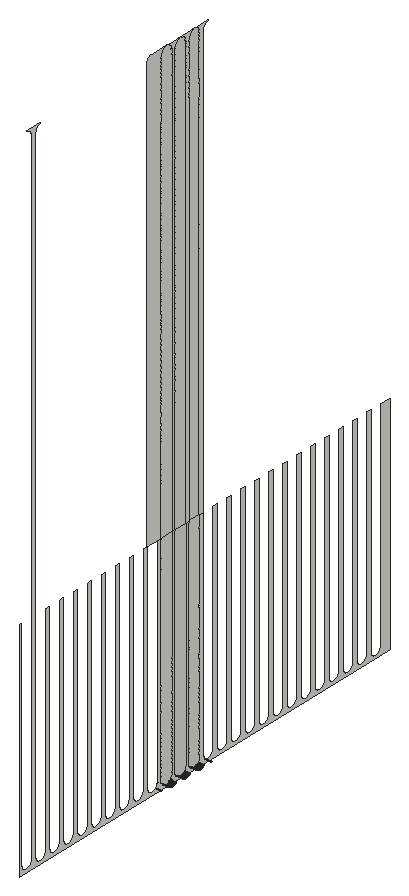
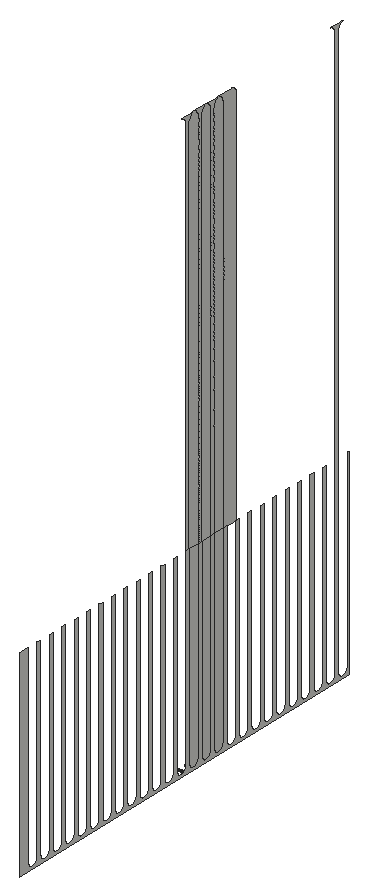
# SketchUp Ruby script. Lengths in inches.
U = 1.inch
M = Sketchup.active_model
def pt(a) = Geom::Point3d.new(a.map { |v| v * U })
def face(e, loops, mat)
  f = e.add_face(loops[0].map { |a| pt(a) })
  loops[1..].each { |l| e.add_face(l.map { |a| pt(a) }).erase! }
  f.material = f.back_material = mat if mat
  f
end
# faces: each face lists its corners as indices into pts; further lists are holes
def faces(e, pts, list, mat = nil) = list.each { |f| face(e, (f[0].is_a?(Array) ? f : [f]).map { |l| l.map { |i| pts[i] } }, mat) }
# xy, xz, yz: faces in a plane at the given z, y or x. An outline is a flat list of corners, or four numbers for a rectangle; further outlines are holes
def ring(l) = l.size == 4 ? [[l[0], l[1]], [l[2], l[1]], [l[2], l[3]], [l[0], l[3]]] : l.each_slice(2).to_a
def flat(e, list, mat, &to3) = list.each { |f| face(e, (f[0].is_a?(Array) ? f : [f]).map { |l| ring(l).map { |u, v| to3.(u, v) } }, mat) }
def xy(e, z, list, mat = nil) = flat(e, list, mat) { |x, y| [x, y, z] }
def xz(e, y, list, mat = nil) = flat(e, list, mat) { |x, z| [x, y, z] }
def yz(e, x, list, mat = nil) = flat(e, list, mat) { |y, z| [x, y, z] }
def lines(e, pts, list) = list.each { |a, b| e.add_line(pt(pts[a]), pt(pts[b])) }
# prism: a flat outline (further loops are holes) pulled along v
def prism(e, loops, v, mat = nil)
  f = face(e, loops, mat); d = Geom::Vector3d.new(v.map { |x| x * U })
  f.pushpull(f.normal.samedirection?(d) ? d.length : -d.length)
end
def box(e, o, s, mat = nil) = prism(e, [[o, [o[0] + s[0], o[1], o[2]], [o[0] + s[0], o[1] + s[1], o[2]], [o[0], o[1] + s[1], o[2]]]], [0, 0, s[2]], mat)
def at(x, y, z, deg = 0) = Geom::Transformation.translation(pt([x, y, z])) * Geom::Transformation.rotation(ORIGIN, Z_AXIS, deg.degrees)
def axes(o, x, y, z) = Geom::Transformation.new([*x, 0, *y, 0, *z, 0, *pt(o).to_a, 1])
def part(name) = M.definitions.add(name)
# library, detail: a bought-in or finely detailed component or shape, given as its bounding box
def library(name, o, s) = part(name).tap { |d| box(d.entities, o, s) }
def detail(e, o, s) = box(e.add_group.entities, o, s)
def put(e, d, t, mat = nil) = e.add_instance(d, t).tap { |i| i.material = mat if mat }
def group(e, t, mat = nil) = e.add_group.tap { |g| g.transformation = t; g.material = mat if mat }.entities
root = M.entities
yz(root,9,[[15,2,88.732,2,88.732,38,87,38,87,3.521,87.003,3.464,87.003,3.407,87,3.363,86.993,3.292,86.983,3.236,86.97,3.18,86.954,3.125,86.936,3.071,86.914,3.018,86.889,2.966,86.862,2.915,86.831,2.867,86.799,2.82,86.763,2.774,86.726,2.731,86.685,2.69,86.643,2.651,86.599,2.615,86.553,2.581,86.504,2.55,86.455,2.521,86.404,2.495,86.351,2.473,86.297,2.452,86.242,2.435,86.187,2.421,86.131,2.41,86.074,2.403,86.017,2.398,85.959,2.396,85.902,2.398,85.845,2.403,85.788,2.41,85.732,2.421,85.676,2.435,85.621,2.452,85.568,2.473,85.515,2.495,85.464,2.521,85.414,2.55,85.366,2.581,85.32,2.615,85.275,2.651,85.233,2.69,85.193,2.731,85.155,2.774,85.12,2.82,85.087,2.867,85.057,2.915,85.029,2.966,85.005,3.018,84.983,3.071,84.964,3.125,84.948,3.18,84.936,3.236,84.926,3.292,84.918,3.363,84.916,3.407,84.916,3.464,84.918,3.521,84.918,38,84.212,38,84.212,3.521,84.215,3.464,84.215,3.407,84.212,3.363,84.205,3.292,84.195,3.236,84.183,3.18,84.167,3.125,84.148,3.071,84.126,3.018,84.102,2.966,84.074,2.915,84.044,2.867,84.011,2.82,83.976,2.774,83.938,2.731,83.898,2.69,83.856,2.651,83.811,2.615,83.765,2.581,83.717,2.55,83.667,2.521,83.616,2.495,83.563,2.473,83.51,2.452,83.455,2.435,83.399,2.421,83.343,2.41,83.286,2.403,83.229,2.398,83.172,2.396,83.114,2.398,83.057,2.403,83,2.41,82.944,2.421,82.889,2.435,82.834,2.452,82.78,2.473,82.727,2.495,82.676,2.521,82.627,2.55,82.578,2.581,82.532,2.615,82.488,2.651,82.446,2.69,82.405,2.731,82.368,2.774,82.332,2.82,82.3,2.867,82.269,2.915,82.242,2.966,82.217,3.018,82.195,3.071,82.177,3.125,82.161,3.18,82.148,3.236,82.138,3.292,82.131,3.363,82.128,3.407,82.128,3.464,82.131,3.521,82.131,38,81.425,38,81.425,3.521,81.428,3.464,81.428,3.407,81.425,3.363,81.418,3.292,81.408,3.236,81.395,3.18,81.379,3.125,81.361,3.071,81.339,3.018,81.314,2.966,81.287,2.915,81.256,2.867,81.224,2.82,81.188,2.774,81.151,2.731,81.11,2.69,81.068,2.651,81.024,2.615,80.978,2.581,80.929,2.55,80.88,2.521,80.829,2.495,80.776,2.473,80.722,2.452,80.667,2.435,80.612,2.421,80.556,2.41,80.499,2.403,80.442,2.398,80.384,2.396,80.327,2.398,80.27,2.403,80.213,2.41,80.157,2.421,80.101,2.435,80.046,2.452,79.993,2.473,79.94,2.495,79.889,2.521,79.839,2.55,79.791,2.581,79.745,2.615,79.7,2.651,79.658,2.69,79.618,2.731,79.58,2.774,79.545,2.82,79.512,2.867,79.482,2.915,79.454,2.966,79.43,3.018,79.408,3.071,79.389,3.125,79.373,3.18,79.361,3.236,79.351,3.292,79.343,3.363,79.341,3.407,79.341,3.464,79.343,3.521,79.343,38,78.637,38,78.637,3.521,78.64,3.464,78.64,3.407,78.637,3.363,78.63,3.292,78.62,3.236,78.608,3.18,78.592,3.125,78.573,3.071,78.551,3.018,78.527,2.966,78.499,2.915,78.469,2.867,78.436,2.82,78.401,2.774,78.363,2.731,78.323,2.69,78.281,2.651,78.236,2.615,78.19,2.581,78.142,2.55,78.092,2.521,78.041,2.495,77.988,2.473,77.935,2.452,77.88,2.435,77.824,2.421,77.768,2.41,77.711,2.403,77.654,2.398,77.597,2.396,77.539,2.398,77.482,2.403,77.425,2.41,77.369,2.421,77.314,2.435,77.259,2.452,77.205,2.473,77.152,2.495,77.101,2.521,77.052,2.55,77.003,2.581,76.957,2.615,76.913,2.651,76.871,2.69,76.83,2.731,76.793,2.774,76.757,2.82,76.725,2.867,76.694,2.915,76.667,2.966,76.642,3.018,76.62,3.071,76.602,3.125,76.586,3.18,76.573,3.236,76.563,3.292,76.556,3.363,76.553,3.407,76.553,3.464,76.556,3.521,76.556,38,75.85,38,75.85,3.521,75.853,3.464,75.853,3.407,75.85,3.363,75.843,3.292,75.833,3.236,75.82,3.18,75.804,3.125,75.786,3.071,75.764,3.018,75.739,2.966,75.712,2.915,75.681,2.867,75.649,2.82,75.613,2.774,75.576,2.731,75.535,2.69,75.493,2.651,75.449,2.615,75.403,2.581,75.354,2.55,75.305,2.521,75.254,2.495,75.201,2.473,75.147,2.452,75.092,2.435,75.037,2.421,74.981,2.41,74.924,2.403,74.867,2.398,74.809,2.396,74.752,2.398,74.695,2.403,74.638,2.41,74.582,2.421,74.526,2.435,74.471,2.452,74.418,2.473,74.365,2.495,74.314,2.521,74.264,2.55,74.216,2.581,74.17,2.615,74.125,2.651,74.083,2.69,74.043,2.731,74.005,2.774,73.97,2.82,73.937,2.867,73.907,2.915,73.879,2.966,73.855,3.018,73.833,3.071,73.814,3.125,73.798,3.18,73.786,3.236,73.776,3.292,73.768,3.363,73.766,3.407,73.766,3.464,73.768,3.521,73.768,38,73.0625,38,73.0625,3.521,73.065,3.464,73.065,3.407,73.0625,3.363,73.055,3.292,73.045,3.236,73.033,3.18,73.017,3.125,72.998,3.071,72.976,3.018,72.952,2.966,72.924,2.915,72.894,2.867,72.861,2.82,72.826,2.774,72.788,2.731,72.748,2.69,72.706,2.651,72.661,2.615,72.615,2.581,72.567,2.55,72.517,2.521,72.466,2.495,72.413,2.473,72.36,2.452,72.305,2.435,72.249,2.421,72.193,2.41,72.136,2.403,72.079,2.398,72.022,2.396,71.964,2.398,71.907,2.403,71.85,2.41,71.794,2.421,71.739,2.435,71.684,2.452,71.63,2.473,71.577,2.495,71.526,2.521,71.477,2.55,71.428,2.581,71.382,2.615,71.338,2.651,71.296,2.69,71.255,2.731,71.218,2.774,71.182,2.82,71.15,2.867,71.119,2.915,71.092,2.966,71.067,3.018,71.045,3.071,71.027,3.125,71.011,3.18,70.998,3.236,70.988,3.292,70.981,3.363,70.978,3.407,70.978,3.464,70.981,3.521,70.981,38,70.275,38,70.275,3.521,70.278,3.464,70.278,3.407,70.275,3.363,70.268,3.292,70.258,3.236,70.245,3.18,70.229,3.125,70.211,3.071,70.189,3.018,70.164,2.966,70.137,2.915,70.106,2.867,70.074,2.82,70.038,2.774,70.001,2.731,69.96,2.69,69.918,2.651,69.874,2.615,69.828,2.581,69.779,2.55,69.73,2.521,69.679,2.495,69.626,2.473,69.572,2.452,69.517,2.435,69.462,2.421,69.406,2.41,69.349,2.403,69.292,2.398,69.234,2.396,69.177,2.398,69.12,2.403,69.063,2.41,69.007,2.421,68.951,2.435,68.896,2.452,68.843,2.473,68.79,2.495,68.739,2.521,68.689,2.55,68.641,2.581,68.595,2.615,68.55,2.651,68.508,2.69,68.468,2.731,68.43,2.774,68.395,2.82,68.362,2.867,68.332,2.915,68.304,2.966,68.28,3.018,68.258,3.071,68.239,3.125,68.223,3.18,68.211,3.236,68.201,3.292,68.193,3.363,68.191,3.407,68.191,3.464,68.193,3.521,68.193,38,67.487,38,67.487,3.521,67.49,3.464,67.49,3.407,67.487,3.363,67.48,3.292,67.47,3.236,67.458,3.18,67.442,3.125,67.423,3.071,67.401,3.018,67.377,2.966,67.349,2.915,67.319,2.867,67.286,2.82,67.251,2.774,67.213,2.731,67.173,2.69,67.131,2.651,67.086,2.615,67.04,2.581,66.992,2.55,66.942,2.521,66.891,2.495,66.838,2.473,66.785,2.452,66.73,2.435,66.674,2.421,66.618,2.41,66.561,2.403,66.504,2.398,66.447,2.396,66.389,2.398,66.332,2.403,66.275,2.41,66.219,2.421,66.164,2.435,66.109,2.452,66.055,2.473,66.002,2.495,65.951,2.521,65.902,2.55,65.853,2.581,65.807,2.615,65.763,2.651,65.721,2.69,65.68,2.731,65.643,2.774,65.607,2.82,65.575,2.867,65.544,2.915,65.517,2.966,65.492,3.018,65.47,3.071,65.452,3.125,65.436,3.18,65.423,3.236,65.413,3.292,65.406,3.363,65.403,3.407,65.403,3.464,65.406,3.521,65.406,38,64.7,38,64.7,3.521,64.703,3.464,64.703,3.407,64.7,3.363,64.693,3.292,64.683,3.236,64.67,3.18,64.654,3.125,64.636,3.071,64.614,3.018,64.589,2.966,64.562,2.915,64.531,2.867,64.499,2.82,64.463,2.774,64.426,2.731,64.385,2.69,64.343,2.651,64.299,2.615,64.253,2.581,64.204,2.55,64.155,2.521,64.104,2.495,64.051,2.473,63.997,2.452,63.942,2.435,63.887,2.421,63.831,2.41,63.774,2.403,63.717,2.398,63.659,2.396,63.602,2.398,63.545,2.403,63.488,2.41,63.432,2.421,63.376,2.435,63.321,2.452,63.268,2.473,63.215,2.495,63.164,2.521,63.114,2.55,63.066,2.581,63.02,2.615,62.975,2.651,62.933,2.69,62.893,2.731,62.855,2.774,62.82,2.82,62.787,2.867,62.757,2.915,62.729,2.966,62.705,3.018,62.683,3.071,62.664,3.125,62.648,3.18,62.636,3.236,62.626,3.292,62.618,3.363,62.616,3.407,62.616,3.464,62.618,3.521,62.618,38,61.912,38,61.912,3.521,61.915,3.464,61.915,3.407,61.912,3.363,61.905,3.292,61.895,3.236,61.883,3.18,61.867,3.125,61.848,3.071,61.826,3.018,61.802,2.966,61.774,2.915,61.744,2.867,61.711,2.82,61.676,2.774,61.638,2.731,61.598,2.69,61.556,2.651,61.511,2.615,61.465,2.581,61.417,2.55,61.367,2.521,61.316,2.495,61.263,2.473,61.21,2.452,61.155,2.435,61.099,2.421,61.043,2.41,60.986,2.403,60.929,2.398,60.872,2.396,60.814,2.398,60.757,2.403,60.7,2.41,60.644,2.421,60.589,2.435,60.534,2.452,60.48,2.473,60.427,2.495,60.376,2.521,60.327,2.55,60.278,2.581,60.232,2.615,60.188,2.651,60.146,2.69,60.105,2.731,60.068,2.774,60.032,2.82,60,2.867,59.969,2.915,59.942,2.966,59.917,3.018,59.895,3.071,59.877,3.125,59.861,3.18,59.848,3.236,59.838,3.292,59.831,3.363,59.828,3.407,59.828,3.464,59.831,3.521,59.831,38,59.125,38,59.125,3.521,59.128,3.464,59.128,3.407,59.125,3.363,59.118,3.292,59.108,3.236,59.095,3.18,59.079,3.125,59.061,3.071,59.039,3.018,59.014,2.966,58.987,2.915,58.956,2.867,58.924,2.82,58.888,2.774,58.851,2.731,58.81,2.69,58.768,2.651,58.724,2.615,58.678,2.581,58.629,2.55,58.58,2.521,58.529,2.495,58.476,2.473,58.422,2.452,58.367,2.435,58.312,2.421,58.256,2.41,58.199,2.403,58.142,2.398,58.084,2.396,58.027,2.398,57.97,2.403,57.913,2.41,57.857,2.421,57.801,2.435,57.746,2.452,57.693,2.473,57.64,2.495,57.589,2.521,57.539,2.55,57.491,2.581,57.445,2.615,57.4,2.651,57.358,2.69,57.318,2.731,57.28,2.774,57.245,2.82,57.212,2.867,57.182,2.915,57.154,2.966,57.13,3.018,57.108,3.071,57.089,3.125,57.073,3.18,57.061,3.236,57.051,3.292,57.043,3.363,57.041,3.407,57.041,3.464,57.043,3.521,57.043,38,56.338,38,56.338,3.521,56.34,3.464,56.34,3.407,56.338,3.363,56.33,3.292,56.32,3.236,56.308,3.18,56.292,3.125,56.273,3.071,56.251,3.018,56.227,2.966,56.199,2.915,56.169,2.867,56.136,2.82,56.101,2.774,56.063,2.731,56.023,2.69,55.981,2.651,55.936,2.615,55.89,2.581,55.842,2.55,55.792,2.521,55.741,2.495,55.688,2.473,55.635,2.452,55.58,2.435,55.524,2.421,55.468,2.41,55.411,2.403,55.354,2.398,55.297,2.396,55.239,2.398,55.182,2.403,55.125,2.41,55.069,2.421,55.014,2.435,54.959,2.452,54.905,2.473,54.852,2.495,54.801,2.521,54.752,2.55,54.703,2.581,54.657,2.615,54.613,2.651,54.571,2.69,54.53,2.731,54.493,2.774,54.457,2.82,54.425,2.867,54.394,2.915,54.367,2.966,54.342,3.018,54.32,3.071,54.302,3.125,54.286,3.18,54.273,3.236,54.263,3.292,54.256,3.363,54.253,3.407,54.253,3.464,54.256,3.521,54.256,38,53.55,38,53.55,3.521,53.553,3.464,53.553,3.407,53.55,3.363,53.543,3.292,53.533,3.236,53.52,3.18,53.504,3.125,53.486,3.071,53.464,3.018,53.439,2.966,53.412,2.915,53.381,2.867,53.349,2.82,53.313,2.774,53.276,2.731,53.235,2.69,53.193,2.651,53.149,2.615,53.103,2.581,53.054,2.55,53.005,2.521,52.954,2.495,52.901,2.473,52.847,2.452,52.792,2.435,52.737,2.421,52.681,2.41,52.624,2.403,52.567,2.398,52.509,2.396,52.452,2.398,52.395,2.403,52.338,2.41,52.282,2.421,52.226,2.435,52.171,2.452,52.118,2.473,52.065,2.495,52.014,2.521,51.964,2.55,51.916,2.581,51.87,2.615,51.825,2.651,51.783,2.69,51.743,2.731,51.705,2.774,51.67,2.82,51.637,2.867,51.607,2.915,51.579,2.966,51.555,3.018,51.533,3.071,51.514,3.125,51.498,3.18,51.486,3.236,51.476,3.292,51.468,3.363,51.466,3.407,51.466,3.464,51.468,3.521,51.468,38,50.762,38,50.762,3.521,50.765,3.464,50.765,3.407,50.762,3.363,50.755,3.292,50.745,3.236,50.733,3.18,50.717,3.125,50.698,3.071,50.676,3.018,50.652,2.966,50.624,2.915,50.594,2.867,50.561,2.82,50.526,2.774,50.488,2.731,50.448,2.69,50.406,2.651,50.361,2.615,50.315,2.581,50.267,2.55,50.217,2.521,50.166,2.495,50.113,2.473,50.06,2.452,50.005,2.435,49.949,2.421,49.893,2.41,49.836,2.403,49.779,2.398,49.722,2.396,49.664,2.398,49.607,2.403,49.55,2.41,49.494,2.421,49.439,2.435,49.384,2.452,49.33,2.473,49.277,2.495,49.226,2.521,49.177,2.55,49.128,2.581,49.082,2.615,49.038,2.651,48.996,2.69,48.955,2.731,48.918,2.774,48.882,2.82,48.85,2.867,48.819,2.915,48.792,2.966,48.767,3.018,48.745,3.071,48.727,3.125,48.711,3.18,48.698,3.236,48.688,3.292,48.681,3.363,48.678,3.407,48.678,3.464,48.681,3.521,48.681,38,47.975,38,47.975,3.521,47.978,3.464,47.978,3.407,47.975,3.363,47.968,3.292,47.958,3.236,47.945,3.18,47.929,3.125,47.911,3.071,47.889,3.018,47.864,2.966,47.837,2.915,47.806,2.867,47.774,2.82,47.738,2.774,47.701,2.731,47.66,2.69,47.618,2.651,47.574,2.615,47.528,2.581,47.479,2.55,47.43,2.521,47.379,2.495,47.326,2.473,47.272,2.452,47.217,2.435,47.162,2.421,47.106,2.41,47.049,2.403,46.992,2.398,46.934,2.396,46.877,2.398,46.82,2.403,46.763,2.41,46.707,2.421,46.651,2.435,46.596,2.452,46.543,2.473,46.49,2.495,46.439,2.521,46.389,2.55,46.341,2.581,46.295,2.615,46.25,2.651,46.208,2.69,46.168,2.731,46.13,2.774,46.095,2.82,46.062,2.867,46.032,2.915,46.004,2.966,45.98,3.018,45.958,3.071,45.939,3.125,45.923,3.18,45.911,3.236,45.901,3.292,45.893,3.363,45.891,3.407,45.891,3.464,45.893,3.521,45.893,38,45.1875,38,45.1875,3.521,45.19,3.464,45.19,3.407,45.1875,3.363,45.18,3.292,45.17,3.236,45.158,3.18,45.142,3.125,45.123,3.071,45.101,3.018,45.077,2.966,45.049,2.915,45.019,2.867,44.986,2.82,44.951,2.774,44.913,2.731,44.873,2.69,44.831,2.651,44.786,2.615,44.74,2.581,44.692,2.55,44.642,2.521,44.591,2.495,44.538,2.473,44.485,2.452,44.43,2.435,44.374,2.421,44.318,2.41,44.261,2.403,44.204,2.398,44.147,2.396,44.089,2.398,44.032,2.403,43.975,2.41,43.919,2.421,43.864,2.435,43.809,2.452,43.755,2.473,43.702,2.495,43.651,2.521,43.602,2.55,43.553,2.581,43.507,2.615,43.463,2.651,43.421,2.69,43.38,2.731,43.343,2.774,43.307,2.82,43.275,2.867,43.244,2.915,43.217,2.966,43.192,3.018,43.17,3.071,43.152,3.125,43.136,3.18,43.123,3.236,43.113,3.292,43.106,3.363,43.103,3.407,43.103,3.464,43.106,3.521,43.106,38,42.4,38,42.4,3.521,42.403,3.464,42.403,3.407,42.4,3.363,42.393,3.292,42.383,3.236,42.37,3.18,42.354,3.125,42.336,3.071,42.314,3.018,42.289,2.966,42.262,2.915,42.231,2.867,42.199,2.82,42.163,2.774,42.126,2.731,42.085,2.69,42.043,2.651,41.999,2.615,41.953,2.581,41.904,2.55,41.855,2.521,41.804,2.495,41.751,2.473,41.697,2.452,41.642,2.435,41.587,2.421,41.531,2.41,41.474,2.403,41.417,2.398,41.359,2.396,41.302,2.398,41.245,2.403,41.188,2.41,41.132,2.421,41.076,2.435,41.021,2.452,40.968,2.473,40.915,2.495,40.864,2.521,40.814,2.55,40.766,2.581,40.72,2.615,40.675,2.651,40.633,2.69,40.593,2.731,40.555,2.774,40.52,2.82,40.487,2.867,40.457,2.915,40.429,2.966,40.405,3.018,40.383,3.071,40.364,3.125,40.348,3.18,40.336,3.236,40.326,3.292,40.318,3.363,40.316,3.407,40.316,3.464,40.318,3.521,40.318,38,39.612,38,39.612,3.521,39.615,3.464,39.615,3.407,39.612,3.363,39.605,3.292,39.595,3.236,39.583,3.18,39.567,3.125,39.548,3.071,39.526,3.018,39.502,2.966,39.474,2.915,39.444,2.867,39.411,2.82,39.376,2.774,39.338,2.731,39.298,2.69,39.256,2.651,39.211,2.615,39.165,2.581,39.117,2.55,39.067,2.521,39.016,2.495,38.963,2.473,38.91,2.452,38.855,2.435,38.799,2.421,38.743,2.41,38.686,2.403,38.629,2.398,38.572,2.396,38.514,2.398,38.457,2.403,38.4,2.41,38.344,2.421,38.289,2.435,38.234,2.452,38.18,2.473,38.127,2.495,38.076,2.521,38.027,2.55,37.978,2.581,37.932,2.615,37.888,2.651,37.846,2.69,37.805,2.731,37.768,2.774,37.732,2.82,37.7,2.867,37.669,2.915,37.642,2.966,37.617,3.018,37.595,3.071,37.577,3.125,37.561,3.18,37.548,3.236,37.538,3.292,37.531,3.363,37.528,3.407,37.528,3.464,37.531,3.521,37.531,38,36.825,38,36.825,3.521,36.828,3.464,36.828,3.407,36.825,3.363,36.818,3.292,36.808,3.236,36.795,3.18,36.779,3.125,36.761,3.071,36.739,3.018,36.714,2.966,36.687,2.915,36.656,2.867,36.624,2.82,36.588,2.774,36.551,2.731,36.51,2.69,36.468,2.651,36.424,2.615,36.378,2.581,36.329,2.55,36.28,2.521,36.229,2.495,36.176,2.473,36.122,2.452,36.067,2.435,36.012,2.421,35.956,2.41,35.899,2.403,35.842,2.398,35.784,2.396,35.727,2.398,35.67,2.403,35.613,2.41,35.557,2.421,35.501,2.435,35.446,2.452,35.393,2.473,35.34,2.495,35.289,2.521,35.239,2.55,35.191,2.581,35.145,2.615,35.1,2.651,35.058,2.69,35.018,2.731,34.98,2.774,34.945,2.82,34.912,2.867,34.882,2.915,34.854,2.966,34.83,3.018,34.808,3.071,34.789,3.125,34.773,3.18,34.761,3.236,34.751,3.292,34.743,3.363,34.741,3.407,34.741,3.464,34.743,3.521,34.743,38,34.037,38,34.037,3.521,34.04,3.464,34.04,3.407,34.037,3.363,34.03,3.292,34.02,3.236,34.008,3.18,33.992,3.125,33.973,3.071,33.951,3.018,33.927,2.966,33.899,2.915,33.869,2.867,33.836,2.82,33.801,2.774,33.763,2.731,33.723,2.69,33.681,2.651,33.636,2.615,33.59,2.581,33.542,2.55,33.492,2.521,33.441,2.495,33.388,2.473,33.335,2.452,33.28,2.435,33.224,2.421,33.168,2.41,33.111,2.403,33.054,2.398,32.997,2.396,32.939,2.398,32.882,2.403,32.825,2.41,32.769,2.421,32.714,2.435,32.659,2.452,32.605,2.473,32.552,2.495,32.501,2.521,32.452,2.55,32.403,2.581,32.357,2.615,32.313,2.651,32.271,2.69,32.23,2.731,32.193,2.774,32.157,2.82,32.125,2.867,32.094,2.915,32.067,2.966,32.042,3.018,32.02,3.071,32.002,3.125,31.986,3.18,31.973,3.236,31.963,3.292,31.956,3.363,31.953,3.407,31.953,3.464,31.956,3.521,31.956,38,31.25,38,31.25,3.521,31.253,3.464,31.253,3.407,31.25,3.363,31.243,3.292,31.233,3.236,31.22,3.18,31.204,3.125,31.186,3.071,31.164,3.018,31.139,2.966,31.112,2.915,31.081,2.867,31.049,2.82,31.013,2.774,30.976,2.731,30.935,2.69,30.893,2.651,30.849,2.615,30.803,2.581,30.754,2.55,30.705,2.521,30.654,2.495,30.601,2.473,30.547,2.452,30.492,2.435,30.437,2.421,30.381,2.41,30.324,2.403,30.267,2.398,30.209,2.396,30.152,2.398,30.095,2.403,30.038,2.41,29.982,2.421,29.926,2.435,29.871,2.452,29.818,2.473,29.765,2.495,29.714,2.521,29.664,2.55,29.616,2.581,29.57,2.615,29.525,2.651,29.483,2.69,29.443,2.731,29.405,2.774,29.37,2.82,29.337,2.867,29.307,2.915,29.279,2.966,29.255,3.018,29.233,3.071,29.214,3.125,29.198,3.18,29.186,3.236,29.176,3.292,29.168,3.363,29.166,3.407,29.166,3.464,29.168,3.521,29.168,38,28.462,38,28.462,3.521,28.465,3.464,28.465,3.407,28.462,3.363,28.455,3.292,28.445,3.236,28.433,3.18,28.417,3.125,28.398,3.071,28.376,3.018,28.352,2.966,28.324,2.915,28.294,2.867,28.261,2.82,28.226,2.774,28.188,2.731,28.148,2.69,28.106,2.651,28.061,2.615,28.015,2.581,27.967,2.55,27.917,2.521,27.866,2.495,27.813,2.473,27.76,2.452,27.705,2.435,27.649,2.421,27.593,2.41,27.536,2.403,27.479,2.398,27.422,2.396,27.364,2.398,27.307,2.403,27.25,2.41,27.194,2.421,27.139,2.435,27.084,2.452,27.03,2.473,26.977,2.495,26.926,2.521,26.877,2.55,26.828,2.581,26.782,2.615,26.738,2.651,26.696,2.69,26.655,2.731,26.618,2.774,26.582,2.82,26.55,2.867,26.519,2.915,26.492,2.966,26.467,3.018,26.445,3.071,26.427,3.125,26.411,3.18,26.398,3.236,26.388,3.292,26.381,3.363,26.378,3.407,26.378,3.464,26.381,3.521,26.381,38,25.675,38,25.675,3.521,25.678,3.464,25.678,3.407,25.675,3.363,25.668,3.292,25.658,3.236,25.645,3.18,25.629,3.125,25.611,3.071,25.589,3.018,25.564,2.966,25.537,2.915,25.506,2.867,25.474,2.82,25.438,2.774,25.401,2.731,25.36,2.69,25.318,2.651,25.274,2.615,25.228,2.581,25.179,2.55,25.13,2.521,25.079,2.495,25.026,2.473,24.972,2.452,24.917,2.435,24.862,2.421,24.806,2.41,24.749,2.403,24.692,2.398,24.634,2.396,24.577,2.398,24.52,2.403,24.463,2.41,24.407,2.421,24.351,2.435,24.296,2.452,24.243,2.473,24.19,2.495,24.139,2.521,24.089,2.55,24.041,2.581,23.995,2.615,23.95,2.651,23.908,2.69,23.868,2.731,23.83,2.774,23.795,2.82,23.762,2.867,23.732,2.915,23.704,2.966,23.68,3.018,23.658,3.071,23.639,3.125,23.623,3.18,23.611,3.236,23.601,3.292,23.593,3.363,23.591,3.407,23.591,3.464,23.593,3.521,23.593,38,22.887,38,22.887,3.521,22.89,3.464,22.89,3.407,22.887,3.363,22.88,3.292,22.87,3.236,22.858,3.18,22.842,3.125,22.823,3.071,22.801,3.018,22.777,2.966,22.749,2.915,22.719,2.867,22.686,2.82,22.651,2.774,22.613,2.731,22.573,2.69,22.531,2.651,22.486,2.615,22.44,2.581,22.392,2.55,22.342,2.521,22.291,2.495,22.238,2.473,22.185,2.452,22.13,2.435,22.074,2.421,22.018,2.41,21.961,2.403,21.904,2.398,21.847,2.396,21.789,2.398,21.732,2.403,21.675,2.41,21.619,2.421,21.564,2.435,21.509,2.452,21.455,2.473,21.402,2.495,21.351,2.521,21.302,2.55,21.253,2.581,21.207,2.615,21.163,2.651,21.121,2.69,21.08,2.731,21.043,2.774,21.007,2.82,20.975,2.867,20.944,2.915,20.917,2.966,20.892,3.018,20.87,3.071,20.852,3.125,20.836,3.18,20.823,3.236,20.813,3.292,20.806,3.363,20.803,3.407,20.803,3.464,20.806,3.521,20.806,38,20.1,38,20.1,3.521,20.103,3.464,20.103,3.407,20.1,3.363,20.093,3.292,20.083,3.236,20.07,3.18,20.054,3.125,20.036,3.071,20.014,3.018,19.989,2.966,19.962,2.915,19.931,2.867,19.899,2.82,19.863,2.774,19.826,2.731,19.785,2.69,19.743,2.651,19.699,2.615,19.653,2.581,19.604,2.55,19.555,2.521,19.504,2.495,19.451,2.473,19.397,2.452,19.342,2.435,19.287,2.421,19.231,2.41,19.174,2.403,19.117,2.398,19.059,2.396,19.002,2.398,18.945,2.403,18.888,2.41,18.832,2.421,18.776,2.435,18.721,2.452,18.668,2.473,18.615,2.495,18.564,2.521,18.514,2.55,18.466,2.581,18.42,2.615,18.375,2.651,18.333,2.69,18.293,2.731,18.255,2.774,18.22,2.82,18.187,2.867,18.157,2.915,18.129,2.966,18.105,3.018,18.083,3.071,18.064,3.125,18.048,3.18,18.036,3.236,18.026,3.292,18.018,3.363,18.016,3.407,18.016,3.464,18.018,3.521,18.018,106.961,18.02,107.015,18.024,107.069,18.031,107.123,18.041,107.177,18.054,107.23,18.069,107.282,18.088,107.334,18.108,107.384,18.132,107.433,18.158,107.481,18.186,107.528,18.217,107.572,18.25,107.616,18.286,107.657,18.323,107.697,18.363,107.734,18.404,107.769,18.448,107.803,18.492,107.834,18.539,107.862,18.587,107.888,18.636,107.911,18.686,107.932,18.738,107.95,18.79,107.966,18.843,107.979,18.896,107.989,18.95,107.996,19.005,108,16.326,108,16.381,107.996,16.435,107.989,16.488,107.979,16.541,107.966,16.593,107.95,16.645,107.932,16.695,107.911,16.744,107.888,16.792,107.862,16.839,107.834,16.883,107.803,16.927,107.769,16.968,107.734,17.008,107.697,17.045,107.657,17.081,107.616,17.114,107.572,17.145,107.528,17.173,107.481,17.199,107.433,17.223,107.384,17.243,107.334,17.262,107.282,17.277,107.23,17.29,107.177,17.3,107.123,17.307,107.069,17.311,107.015,17.3125,106.961,17.3125,3.521,17.315,3.464,17.315,3.407,17.3125,3.363,17.305,3.292,17.295,3.236,17.283,3.18,17.267,3.125,17.248,3.071,17.226,3.018,17.202,2.966,17.174,2.915,17.144,2.867,17.111,2.82,17.076,2.774,17.038,2.731,16.998,2.69,16.956,2.651,16.911,2.615,16.865,2.581,16.817,2.55,16.767,2.521,16.716,2.495,16.663,2.473,16.61,2.452,16.555,2.435,16.499,2.421,16.443,2.41,16.386,2.403,16.329,2.398,16.272,2.396,16.214,2.398,16.157,2.403,16.1,2.41,16.044,2.421,15.989,2.435,15.934,2.452,15.88,2.473,15.827,2.495,15.776,2.521,15.727,2.55,15.678,2.581,15.632,2.615,15.588,2.651,15.546,2.69,15.505,2.731,15.468,2.774,15.432,2.82,15.4,2.867,15.369,2.915,15.342,2.966,15.317,3.018,15.295,3.071,15.277,3.125,15.261,3.18,15.248,3.236,15.238,3.292,15.231,3.363,15.228,3.407,15.228,3.464,15.231,3.521,15.231,38,15,38],[44.147,2.396,44.204,2.398,44.261,2.403,44.318,2.41,44.374,2.421,44.43,2.435,44.485,2.452,44.538,2.473,44.591,2.495,44.642,2.521,44.692,2.55,44.74,2.581,44.786,2.615,44.831,2.651,44.873,2.69,44.913,2.731,44.951,2.774,44.986,2.82,45.019,2.867,45.049,2.915,45.077,2.966,45.101,3.018,45.123,3.071,45.142,3.125,45.158,3.18,45.17,3.236,45.18,3.292,45.1875,3.363,45.1875,38,43.106,38,43.106,3.363,43.113,3.292,43.123,3.236,43.136,3.18,43.152,3.125,43.17,3.071,43.192,3.018,43.217,2.966,43.244,2.915,43.275,2.867,43.307,2.82,43.343,2.774,43.38,2.731,43.421,2.69,43.463,2.651,43.507,2.615,43.553,2.581,43.602,2.55,43.651,2.521,43.702,2.495,43.755,2.473,43.809,2.452,43.864,2.435,43.919,2.421,43.975,2.41,44.032,2.403,44.089,2.398],[46.934,2.396,46.992,2.398,47.049,2.403,47.106,2.41,47.162,2.421,47.217,2.435,47.272,2.452,47.326,2.473,47.379,2.495,47.43,2.521,47.479,2.55,47.528,2.581,47.574,2.615,47.618,2.651,47.66,2.69,47.701,2.731,47.738,2.774,47.774,2.82,47.806,2.867,47.837,2.915,47.864,2.966,47.889,3.018,47.911,3.071,47.929,3.125,47.945,3.18,47.958,3.236,47.968,3.292,47.975,3.363,47.975,38,45.893,38,45.893,3.363,45.901,3.292,45.911,3.236,45.923,3.18,45.939,3.125,45.958,3.071,45.98,3.018,46.004,2.966,46.032,2.915,46.062,2.867,46.095,2.82,46.13,2.774,46.168,2.731,46.208,2.69,46.25,2.651,46.295,2.615,46.341,2.581,46.389,2.55,46.439,2.521,46.49,2.495,46.543,2.473,46.596,2.452,46.651,2.435,46.707,2.421,46.763,2.41,46.82,2.403,46.877,2.398],[49.722,2.396,49.779,2.398,49.836,2.403,49.893,2.41,49.949,2.421,50.005,2.435,50.06,2.452,50.113,2.473,50.166,2.495,50.217,2.521,50.267,2.55,50.315,2.581,50.361,2.615,50.406,2.651,50.448,2.69,50.488,2.731,50.526,2.774,50.561,2.82,50.594,2.867,50.624,2.915,50.652,2.966,50.676,3.018,50.698,3.071,50.717,3.125,50.733,3.18,50.745,3.236,50.755,3.292,50.762,3.363,50.762,38,48.681,38,48.681,3.363,48.688,3.292,48.698,3.236,48.711,3.18,48.727,3.125,48.745,3.071,48.767,3.018,48.792,2.966,48.819,2.915,48.85,2.867,48.882,2.82,48.918,2.774,48.955,2.731,48.996,2.69,49.038,2.651,49.082,2.615,49.128,2.581,49.177,2.55,49.226,2.521,49.277,2.495,49.33,2.473,49.384,2.452,49.439,2.435,49.494,2.421,49.55,2.41,49.607,2.403,49.664,2.398],[42.4,3.363,42.403,3.407,42.403,3.464,42.4,3.521],
  [43.106,3.363,43.106,3.521,43.103,3.464,43.103,3.407],[45.1875,3.363,45.19,3.407,45.19,3.464,45.1875,3.521],[45.893,3.363,45.893,3.521,45.891,3.464,45.891,3.407],[47.975,3.363,47.978,3.407,47.978,3.464,47.975,3.521],[48.681,3.363,48.681,3.521,48.678,3.464,48.678,3.407],
  [50.762,3.363,50.765,3.407,50.765,3.464,50.762,3.521],[51.468,3.363,51.468,3.521,51.466,3.464,51.466,3.407],[40.318,38,43.106,38,43.106,106.961,43.107,107.015,43.112,107.069,43.119,107.123,43.129,107.177,43.141,107.23,43.157,107.282,43.175,107.334,43.196,107.384,43.219,107.433,43.245,107.481,43.274,107.528,43.305,107.572,43.338,107.616,43.373,107.657,43.411,107.697,43.45,107.734,43.492,107.769,43.535,107.803,43.58,107.834,43.626,107.862,43.674,107.888,43.723,107.911,43.774,107.932,43.825,107.95,43.877,107.966,43.93,107.979,43.984,107.989,44.038,107.996,44.092,108,41.305,108,41.25,107.996,41.196,107.989,41.143,107.979,41.09,107.966,41.038,107.95,40.986,107.932,40.936,107.911,40.887,107.888,40.839,107.862,40.792,107.834,40.748,107.803,40.704,107.769,40.663,107.734,40.623,107.697,40.586,107.657,40.55,107.616,40.517,107.572,40.486,107.528,40.458,107.481,40.432,107.433,40.408,107.384,40.388,107.334,40.369,107.282,40.354,107.23,40.341,107.177,40.331,107.123,40.324,107.069,40.32,107.015,40.318,106.961],[43.106,38,45.1875,38,45.1875,106.961,45.186,107.015,45.182,107.069,45.175,107.123,45.165,107.177,45.152,107.23,45.137,107.282,45.118,107.334,45.098,107.384,45.074,107.433,45.048,107.481,45.02,107.528,44.989,107.572,44.956,107.616,44.92,107.657,44.883,107.697,44.843,107.734,44.802,107.769,44.758,107.803,44.714,107.834,44.667,107.862,44.619,107.888,44.57,107.911,44.52,107.932,44.468,107.95,44.416,107.966,44.363,107.979,44.31,107.989,44.256,107.996,44.201,108,44.092,108,44.038,107.996,43.984,107.989,43.93,107.979,43.877,107.966,43.825,107.95,43.774,107.932,43.723,107.911,43.674,107.888,43.626,107.862,43.58,107.834,43.535,107.803,43.492,107.769,43.45,107.734,43.411,107.697,43.373,107.657,43.338,107.616,43.305,107.572,43.274,107.528,43.245,107.481,43.219,107.433,43.196,107.384,43.175,107.334,43.157,107.282,43.141,107.23,43.129,107.177,43.119,107.123,43.112,107.069,43.107,107.015,43.106,106.961],[45.1875,38,45.893,38,45.893,106.961,45.895,107.015,45.899,107.069,45.906,107.123,45.916,107.177,45.929,107.23,45.944,107.282,45.963,107.334,45.983,107.384,46.007,107.433,46.033,107.481,46.061,107.528,46.092,107.572,46.125,107.616,46.161,107.657,46.198,107.697,46.238,107.734,46.279,107.769,46.323,107.803,46.367,107.834,46.414,107.862,46.462,107.888,46.511,107.911,46.561,107.932,46.613,107.95,46.665,107.966,46.718,107.979,46.771,107.989,46.825,107.996,46.88,108,44.201,108,44.256,107.996,44.31,107.989,44.363,107.979,44.416,107.966,44.468,107.95,44.52,107.932,44.57,107.911,44.619,107.888,44.667,107.862,44.714,107.834,44.758,107.803,44.802,107.769,44.843,107.734,44.883,107.697,44.92,107.657,44.956,107.616,44.989,107.572,45.02,107.528,45.048,107.481,45.074,107.433,45.098,107.384,45.118,107.334,45.137,107.282,45.152,107.23,45.165,107.177,45.175,107.123,45.182,107.069,45.186,107.015,45.1875,106.961],
  [45.893,38,47.975,38,47.975,106.961,47.974,107.015,47.969,107.069,47.962,107.123,47.952,107.177,47.94,107.23,47.924,107.282,47.906,107.334,47.885,107.384,47.862,107.433,47.836,107.481,47.807,107.528,47.776,107.572,47.743,107.616,47.708,107.657,47.67,107.697,47.631,107.734,47.589,107.769,47.546,107.803,47.501,107.834,47.455,107.862,47.407,107.888,47.358,107.911,47.307,107.932,47.256,107.95,47.204,107.966,47.151,107.979,47.097,107.989,47.043,107.996,46.989,108,46.88,108,46.825,107.996,46.771,107.989,46.718,107.979,46.665,107.966,46.613,107.95,46.561,107.932,46.511,107.911,46.462,107.888,46.414,107.862,46.367,107.834,46.323,107.803,46.279,107.769,46.238,107.734,46.198,107.697,46.161,107.657,46.125,107.616,46.092,107.572,46.061,107.528,46.033,107.481,46.007,107.433,45.983,107.384,45.963,107.334,45.944,107.282,45.929,107.23,45.916,107.177,45.906,107.123,45.899,107.069,45.895,107.015,45.893,106.961],[47.975,38,48.681,38,48.681,106.961,48.682,107.015,48.687,107.069,48.694,107.123,48.704,107.177,48.716,107.23,48.732,107.282,48.75,107.334,48.771,107.384,48.794,107.433,48.82,107.481,48.849,107.528,48.88,107.572,48.913,107.616,48.948,107.657,48.986,107.697,49.025,107.734,49.067,107.769,49.11,107.803,49.155,107.834,49.201,107.862,49.249,107.888,49.298,107.911,49.349,107.932,49.4,107.95,49.452,107.966,49.505,107.979,49.559,107.989,49.613,107.996,49.667,108,46.989,108,47.043,107.996,47.097,107.989,47.151,107.979,47.204,107.966,47.256,107.95,47.307,107.932,47.358,107.911,47.407,107.888,47.455,107.862,47.501,107.834,47.546,107.803,47.589,107.769,47.631,107.734,47.67,107.697,47.708,107.657,47.743,107.616,47.776,107.572,47.807,107.528,47.836,107.481,47.862,107.433,47.885,107.384,47.906,107.334,47.924,107.282,47.94,107.23,47.952,107.177,47.962,107.123,47.969,107.069,47.974,107.015,47.975,106.961],[48.681,38,50.762,38,50.762,106.961,50.761,107.015,50.757,107.069,50.75,107.123,50.74,107.177,50.727,107.23,50.712,107.282,50.693,107.334,50.673,107.384,50.649,107.433,50.623,107.481,50.595,107.528,50.564,107.572,50.531,107.616,50.495,107.657,50.458,107.697,50.418,107.734,50.377,107.769,50.333,107.803,50.289,107.834,50.242,107.862,50.194,107.888,50.145,107.911,50.095,107.932,50.043,107.95,49.991,107.966,49.938,107.979,49.885,107.989,49.831,107.996,49.776,108,49.667,108,49.613,107.996,49.559,107.989,49.505,107.979,49.452,107.966,49.4,107.95,49.349,107.932,49.298,107.911,49.249,107.888,49.201,107.862,49.155,107.834,49.11,107.803,49.067,107.769,49.025,107.734,48.986,107.697,48.948,107.657,48.913,107.616,48.88,107.572,48.849,107.528,48.82,107.481,48.794,107.433,48.771,107.384,48.75,107.334,48.732,107.282,48.716,107.23,48.704,107.177,48.694,107.123,48.687,107.069,48.682,107.015,48.681,106.961],[50.762,38,51.468,38,51.468,106.961,51.47,107.015,51.474,107.069,51.481,107.123,51.491,107.177,51.504,107.23,51.519,107.282,51.538,107.334,51.558,107.384,51.582,107.433,51.608,107.481,51.636,107.528,51.667,107.572,51.7,107.616,51.736,107.657,51.773,107.697,51.813,107.734,51.854,107.769,51.898,107.803,51.942,107.834,51.989,107.862,52.037,107.888,52.086,107.911,52.136,107.932,52.1875,107.95,52.24,107.966,52.293,107.979,52.346,107.989,52.4,107.996,52.455,108,49.776,108,49.831,107.996,49.885,107.989,49.938,107.979,49.991,107.966,50.043,107.95,50.095,107.932,50.145,107.911,50.194,107.888,50.242,107.862,50.289,107.834,50.333,107.803,50.377,107.769,50.418,107.734,50.458,107.697,50.495,107.657,50.531,107.616,50.564,107.572,50.595,107.528,50.623,107.481,50.649,107.433,50.673,107.384,50.693,107.334,50.712,107.282,50.727,107.23,50.74,107.177,50.75,107.123,50.757,107.069,50.761,107.015,50.762,106.961]])
p = [[9,43.809,2.452],[9,43.864,2.435],[10,43.864,2.435],[10,43.809,2.452],[9,43.919,2.421],[10,43.919,2.421],
  [9,43.975,2.41],[10,43.975,2.41],[9,44.032,2.403],[10,44.032,2.403],[9,44.089,2.398],[10,44.089,2.398],
  [9,44.147,2.396],[10,44.147,2.396],[9,44.204,2.398],[10,44.204,2.398],[9,44.261,2.403],[10,44.261,2.403],
  [9,44.318,2.41],[10,44.318,2.41],[9,44.374,2.421],[10,44.374,2.421],[9,44.43,2.435],[10,44.43,2.435],
  [9,44.485,2.452],[10,44.485,2.452],[9,46.596,2.452],[9,46.651,2.435],[10,46.651,2.435],[10,46.596,2.452],
  [9,46.707,2.421],[10,46.707,2.421],[9,46.763,2.41],[10,46.763,2.41],[9,46.82,2.403],[10,46.82,2.403],
  [9,46.877,2.398],[10,46.877,2.398],[9,46.934,2.396],[10,46.934,2.396],[9,46.992,2.398],[10,46.992,2.398],
  [9,47.049,2.403],[10,47.049,2.403],[9,47.106,2.41],[10,47.106,2.41],[9,47.162,2.421],[10,47.162,2.421],
  [9,47.217,2.435],[10,47.217,2.435],[9,47.272,2.452],[10,47.272,2.452],[9,49.384,2.452],[9,49.439,2.435],
  [10,49.439,2.435],[10,49.384,2.452],[9,49.494,2.421],[10,49.494,2.421],[9,49.55,2.41],[10,49.55,2.41],
  [9,49.607,2.403],[10,49.607,2.403],[9,49.664,2.398],[10,49.664,2.398],[9,49.722,2.396],[10,49.722,2.396],
  [9,49.779,2.398],[10,49.779,2.398],[9,49.836,2.403],[10,49.836,2.403],[9,49.893,2.41],[10,49.893,2.41],
  [9,49.949,2.421],[10,49.949,2.421],[9,50.005,2.435],[10,50.005,2.435],[9,50.06,2.452],[10,50.06,2.452],
  [9,43.553,2.581],[9,43.602,2.55],[10,43.602,2.55],[10,43.553,2.581],[9,43.651,2.521],[10,43.651,2.521],
  [9,43.702,2.495],[10,43.702,2.495],[9,43.755,2.473],[10,43.755,2.473],[9,44.538,2.473],[10,44.538,2.473],
  [9,44.591,2.495],[10,44.591,2.495],[9,44.642,2.521],[10,44.642,2.521],[9,44.692,2.55],[10,44.692,2.55],
  [9,44.74,2.581],[10,44.74,2.581],[9,46.341,2.581],[9,46.389,2.55],[10,46.389,2.55],[10,46.341,2.581],
  [9,46.439,2.521],[10,46.439,2.521],[9,46.49,2.495],[10,46.49,2.495],[9,46.543,2.473],[10,46.543,2.473],
  [9,47.326,2.473],[10,47.326,2.473],[9,47.379,2.495],[10,47.379,2.495],[9,47.43,2.521],[10,47.43,2.521],
  [9,47.479,2.55],[10,47.479,2.55],[9,47.528,2.581],[10,47.528,2.581],[9,49.128,2.581],[9,49.177,2.55],
  [10,49.177,2.55],[10,49.128,2.581],[9,49.226,2.521],[10,49.226,2.521],[9,49.277,2.495],[10,49.277,2.495],
  [9,49.33,2.473],[10,49.33,2.473],[9,50.113,2.473],[10,50.113,2.473],[9,50.166,2.495],[10,50.166,2.495],
  [9,50.217,2.521],[10,50.217,2.521],[9,50.267,2.55],[10,50.267,2.55],[9,50.315,2.581],[10,50.315,2.581],
  [9,51.916,2.581],[9,51.964,2.55],[10,51.964,2.55],[10,51.916,2.581],[9,52.014,2.521],[10,52.014,2.521],
  [9,43.463,2.651],[9,43.507,2.615],[10,43.507,2.615],[10,43.463,2.651],[9,44.786,2.615],[10,44.786,2.615],
  [9,44.831,2.651],[10,44.831,2.651],[9,46.25,2.651],[9,46.295,2.615],[10,46.295,2.615],[10,46.25,2.651],
  [9,47.574,2.615],[10,47.574,2.615],[9,47.618,2.651],[10,47.618,2.651],[9,49.038,2.651],[9,49.082,2.615],
  [10,49.082,2.615],[10,49.038,2.651],[9,50.361,2.615],[10,50.361,2.615],[9,50.406,2.651],[10,50.406,2.651],
  [9,51.825,2.651],[9,51.87,2.615],[10,51.87,2.615],[10,51.825,2.651],[9,42.043,2.651],[9,42.085,2.69],
  [10,42.085,2.69],[10,42.043,2.651],[9,42.126,2.731],[10,42.126,2.731],[9,43.421,2.69],[10,43.421,2.69],
  [9,44.873,2.69],[10,44.873,2.69],[9,44.913,2.731],[10,44.913,2.731],[9,46.208,2.69],[10,46.208,2.69],
  [9,47.66,2.69],[10,47.66,2.69],[9,47.701,2.731],[10,47.701,2.731],[9,48.996,2.69],[10,48.996,2.69],
  [9,50.448,2.69],[10,50.448,2.69],[9,50.488,2.731],[10,50.488,2.731],[9,51.783,2.69],[10,51.783,2.69],
  [9,42.4,38],[9,42.4,39.466]]
faces(root,p,[[0,1,2,3],[1,4,5,2],[4,6,7,5],[6,8,9,7],[8,10,11,9],[10,12,13,11],[12,14,15,13],[14,16,17,15],
  [16,18,19,17],[18,20,21,19],[20,22,23,21],[22,24,25,23],[26,27,28,29],[27,30,31,28],[30,32,33,31],[32,34,35,33],
  [34,36,37,35],[36,38,39,37],[38,40,41,39],[40,42,43,41],[42,44,45,43],[44,46,47,45],[46,48,49,47],[48,50,51,49],
  [52,53,54,55],[53,56,57,54],[56,58,59,57],[58,60,61,59],[60,62,63,61],[62,64,65,63],[64,66,67,65],[66,68,69,67],
  [68,70,71,69],[70,72,73,71],[72,74,75,73],[74,76,77,75],[78,79,80,81],[79,82,83,80],[82,84,85,83],[84,86,87,85],
  [86,0,3,87],[24,88,89,25],[88,90,91,89],[90,92,93,91],[92,94,95,93],[94,96,97,95],[98,99,100,101],[99,102,103,100],
  [102,104,105,103],[104,106,107,105],[106,26,29,107],[50,108,109,51],[108,110,111,109],[110,112,113,111],[112,114,115,113],[114,116,117,115],
  [118,119,120,121],[119,122,123,120],[122,124,125,123],[124,126,127,125],[126,52,55,127],[76,128,129,77],[128,130,131,129],[130,132,133,131],
  [132,134,135,133],[134,136,137,135],[138,139,140,141],[139,142,143,140],[144,145,146,147],[145,78,81,146],[96,148,149,97],[148,150,151,149],
  [152,153,154,155],[153,98,101,154],[116,156,157,117],[156,158,159,157],[160,161,162,163],[161,118,121,162],[136,164,165,137],[164,166,167,165],
  [168,169,170,171],[169,138,141,170],[172,173,174,175],[173,176,177,174],[178,144,147,179],[150,180,181,151],[180,182,183,181],[184,152,155,185],
  [158,186,187,159],[186,188,189,187],[190,160,163,191],[166,192,193,167],[192,194,195,193],[196,168,171,197]])
lines(root,p,[[198,199]])
